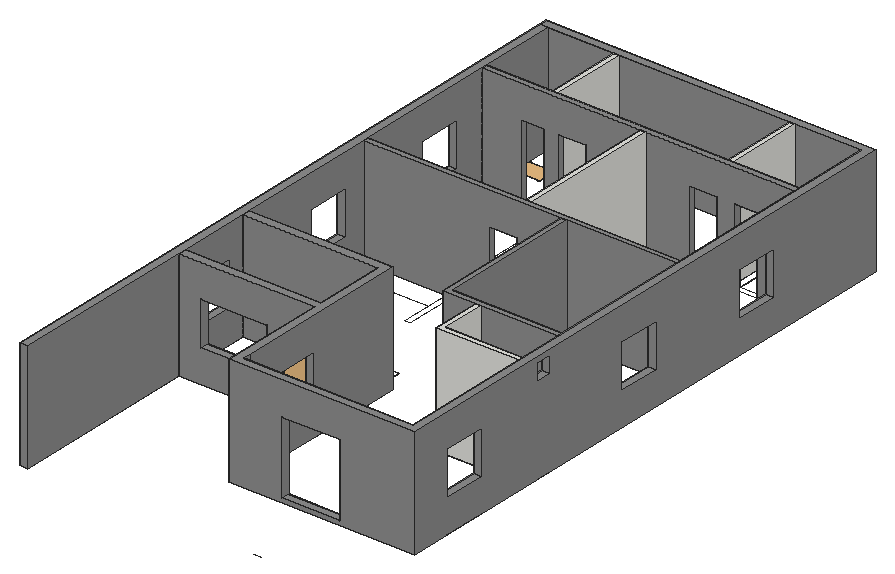
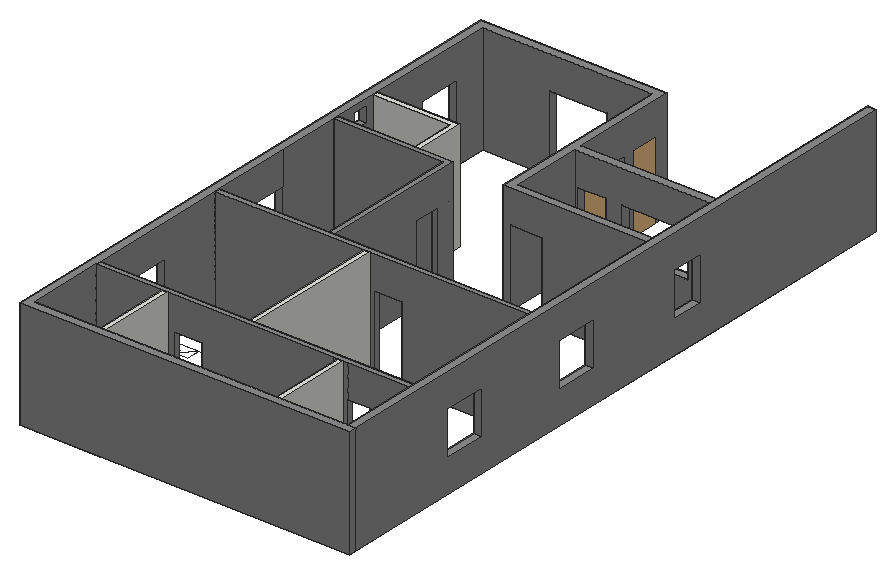
# SketchUp Ruby script. Lengths in inches.
U = 1.inch
M = Sketchup.active_model
def pt(a) = Geom::Point3d.new(a.map { |v| v * U })
def face(e, loops, mat)
  f = e.add_face(loops[0].map { |a| pt(a) })
  loops[1..].each { |l| e.add_face(l.map { |a| pt(a) }).erase! }
  f.material = f.back_material = mat if mat
  f
end
# faces: each face lists its corners as indices into pts; further lists are holes
def faces(e, pts, list, mat = nil) = list.each { |f| face(e, (f[0].is_a?(Array) ? f : [f]).map { |l| l.map { |i| pts[i] } }, mat) }
# xy, xz, yz: faces in a plane at the given z, y or x. An outline is a flat list of corners, or four numbers for a rectangle; further outlines are holes
def ring(l) = l.size == 4 ? [[l[0], l[1]], [l[2], l[1]], [l[2], l[3]], [l[0], l[3]]] : l.each_slice(2).to_a
def flat(e, list, mat, &to3) = list.each { |f| face(e, (f[0].is_a?(Array) ? f : [f]).map { |l| ring(l).map { |u, v| to3.(u, v) } }, mat) }
def xy(e, z, list, mat = nil) = flat(e, list, mat) { |x, y| [x, y, z] }
def xz(e, y, list, mat = nil) = flat(e, list, mat) { |x, z| [x, y, z] }
def yz(e, x, list, mat = nil) = flat(e, list, mat) { |y, z| [x, y, z] }
def lines(e, pts, list) = list.each { |a, b| e.add_line(pt(pts[a]), pt(pts[b])) }
# prism: a flat outline (further loops are holes) pulled along v
def prism(e, loops, v, mat = nil)
  f = face(e, loops, mat); d = Geom::Vector3d.new(v.map { |x| x * U })
  f.pushpull(f.normal.samedirection?(d) ? d.length : -d.length)
end
def box(e, o, s, mat = nil) = prism(e, [[o, [o[0] + s[0], o[1], o[2]], [o[0] + s[0], o[1] + s[1], o[2]], [o[0], o[1] + s[1], o[2]]]], [0, 0, s[2]], mat)
def at(x, y, z, deg = 0) = Geom::Transformation.translation(pt([x, y, z])) * Geom::Transformation.rotation(ORIGIN, Z_AXIS, deg.degrees)
def axes(o, x, y, z) = Geom::Transformation.new([*x, 0, *y, 0, *z, 0, *pt(o).to_a, 1])
def part(name) = M.definitions.add(name)
# library, detail: a bought-in or finely detailed component or shape, given as its bounding box
def library(name, o, s) = part(name).tap { |d| box(d.entities, o, s) }
def detail(e, o, s) = box(e.add_group.entities, o, s)
def put(e, d, t, mat = nil) = e.add_instance(d, t).tap { |i| i.material = mat if mat }
def group(e, t, mat = nil) = e.add_group.tap { |g| g.transformation = t; g.material = mat if mat }.entities
root = M.entities
M.materials.add("[Color M04]").color = [142, 142, 142]
c1 = library("PINTU 6 YA",[0,-0.6875,0],[35.83,8.07,80.71])
c2 = part("*U6")
p = [[-20,-17,0],[-20,23,0],[-18.25,23,0],[-18.25,-17,0],[20,-17,0],[19.92,-14.49,0],
  [19.68,-11.99,0],[19.29,-9.5,0],[18.74,-7.05,0],[18.04,-4.64,0],[17.19,-2.28,0],[16.19,0.03,0],
  [15.05,2.27,0],[13.77,4.43,0],[12.36,6.51,0],[10.82,8.5,0],[9.16,10.38,0],[7.38,12.16,0],
  [5.5,13.82,0],[3.51,15.36,0],[1.43,16.77,0],[-0.73,18.05,0],[-2.97,19.19,0],[-5.28,20.19,0],
  [-7.64,21.04,0],[-10.05,21.74,0],[-12.5,22.29,0],[-14.99,22.68,0],[-17.49,22.92,0],[-20,-23,0],
  [20,-23,0]]
lines(c2.entities,p,[[0,1],[1,2],[2,3],[3,0],[4,5],[5,6],[6,7],[7,8],[8,9],[9,10],[10,11],[11,12],
  [12,13],[13,14],[14,15],[15,16],[16,17],[17,18],[18,19],[19,20],[20,21],[21,22],[22,23],[23,24],
  [24,25],[25,26],[26,27],[27,28],[28,1],[0,29],[4,30]])
c3 = part("new block 03")
p = [[-4.5,18,0],[4.5,18,0],[4.5,-18,0],[-4.5,-18,0],[-1.33,-18,0],[-1.33,18,0],
  [1.57,18,0],[1.57,-18,0]]
lines(c3.entities,p,[[0,1],[1,2],[2,3],[3,0],[4,5],[5,6],[6,7]])
c4 = part("VENTILATOR")
p = [[-4.5,8.5,0],[4.5,8.5,0],[4.5,-8.5,0],[-4.5,-8.5,0],[0.58,8.5,0],[0.58,-8.5,0],
  [0,-8.5,0],[-1.15,-8.5,0],[-0.58,-8.5,0],[-0.58,8.5,0],[-1.15,8.5,0],[0,8.5,0]]
lines(c4.entities,p,[[0,1],[1,2],[2,3],[3,0],[4,5],[6,7],[8,9],[10,11]])
c5 = part("Bed - Queen")
p = [[22,23.6,0],[16.8,23.6,0],[22,38.8,0],[1.2,38.8,0],[1.2,25.6,0],[-1.2,38.8,0],
  [-1.2,25.6,0],[-22,38.8,0],[-22,25.6,0],[30,-40,0],[-30,-40,0],[-30,40,0],
  [14.8,23.2,0],[-30,23.2,0],[-30,25.6,0],[14.8,25.6,0],[30,40,0],[30,10.4,0],
  [14.8,10.4,0]]
lines(c5.entities,p,[[0,1],[2,0],[3,2],[4,3],[5,6],[7,5],[8,7],[9,10],[10,11],[12,13],[14,15],[11,16],
  [16,9],[17,15],[18,17],[15,18]])
c6 = library("*U4",[-21.75,-41.51,0],[21,28.01,0.01])
c7 = library("SINK",[-14.49,-22.42,0],[28.98,44.84,0.01])
c8 = part("new block 02")
p = [[-4.5,24,0],[4.5,24,0],[4.5,-24,0],[-4.5,-24,0],[-0.96,24,0],[-0.96,-24,0],
  [1.12,-24,0],[1.12,24,0]]
lines(c8.entities,p,[[0,1],[1,2],[2,3],[3,0],[4,5],[5,6],[6,7]])
c9 = part("Group14\#1")
box(c9.entities,[324.26,626,0],[6,84,120])
c10 = part("Group16\#1")
box(c10.entities,[132.26,626,0],[6,84,120])
c11 = part("Group20\#1")
box(c11.entities,[233.26,464,0],[6,156,120])
c12 = part("Group25\#1")
xy(c12.entities,0,[[312.3125,242,312.3125,265.39,318.3125,265.39,318.3125,248,402.3125,248,402.3125,242],[312.3125,289.39,318.3125,296]])
xy(c12.entities,84,[[312.3125,265.39,318.3125,289.39]])
xy(c12.entities,120,[[312.3125,242,402.3125,242,402.3125,248,318.3125,248,318.3125,296,312.3125,296]])
xz(c12.entities,242,[[312.3125,0,402.3125,120]])
xz(c12.entities,248,[[318.3125,0,402.3125,120]])
xz(c12.entities,265.39,[[312.3125,0,318.3125,84]])
xz(c12.entities,289.39,[[312.3125,0,318.3125,84]])
xz(c12.entities,296,[[312.3125,0,318.3125,120]])
yz(c12.entities,312.3125,[[242,0,242,120,296,120,296,0,289.39,0,289.39,84,265.39,84,265.39,0]])
yz(c12.entities,318.3125,[[248,0,265.39,0,265.39,84,289.39,84,289.39,0,296,0,296,120,248,120]])
yz(c12.entities,402.3125,[[242,0,248,120]])
p = [[11.9,753.72,126],[11.75,753.71,126],[14.46,751.33,126],[14.46,751.48,126],[14.44,751.64,126],[14.42,751.79,126],
  [14.38,751.95,126],[14.33,752.1,126],[14.28,752.25,126],[14.21,752.39,126],[14.14,752.53,126],[14.06,752.66,126],
  [13.97,752.79,126],[13.87,752.91,126],[13.76,753.02,126],[13.64,753.13,126],[13.52,753.23,126],[13.39,753.32,126],
  [13.26,753.41,126],[13.125,753.48,126],[12.98,753.54,126],[12.83,753.6,126],[12.68,753.65,126],[12.53,753.68,126],
  [12.375,753.71,126],[12.22,753.72,126],[12.0625,753.73,126],[11.59,753.68,126],[11.44,753.65,126],[11.29,753.6,126],
  [11.14,753.54,126],[11,753.48,126],[10.86,753.41,126],[10.73,753.32,126],[10.6,753.23,126],[10.48,753.13,126],
  [10.36,753.02,126],[10.26,752.91,126],[10.16,752.79,126],[10.07,752.66,126],[9.98,752.53,126],[9.91,752.39,126],
  [9.84,752.25,126],[9.79,752.1,126],[9.74,751.95,126],[9.71,751.79,126],[9.68,751.64,126],[9.67,751.48,126],
  [9.66,751.33,126],[9.67,751.17,126],[9.68,751.01,126],[9.71,750.86,126],[9.74,750.71,126],[9.79,750.55,126],
  [9.84,750.41,126],[9.91,750.26,126],[9.98,750.125,126],[10.07,749.99,126],[10.16,749.87,126],[10.26,749.74,126],
  [10.36,749.63,126],[10.48,749.52,126],[10.6,749.42,126],[10.73,749.33,126],[10.86,749.25,126],[11,749.17,126],
  [11.14,749.11,126],[11.29,749.05,126],[11.44,749.01,126],[11.59,748.97,126],[11.75,748.95,126],[11.9,748.93,126],
  [12.0625,748.93,126],[12.22,748.93,126],[12.375,748.95,126],[12.53,748.97,126],[12.68,749.01,126],[12.83,749.05,126],
  [12.98,749.11,126],[13.125,749.17,126],[13.26,749.25,126],[13.39,749.33,126],[13.52,749.42,126],[13.64,749.52,126],
  [13.76,749.63,126],[13.87,749.74,126],[13.97,749.87,126],[14.06,749.99,126],[14.14,750.125,126],[14.21,750.26,126],
  [14.28,750.41,126],[14.33,750.55,126],[14.38,750.71,126],[14.42,750.86,126],[14.44,751.01,126],[14.46,751.17,126],
  [166.65,162.5,126],[169.72,164.68,126],[166.65,167.26,126],[245.95,56.1875,120],[254.15,56.1875,120]]
lines(root,p,[[0,1],[2,3],[3,4],[4,5],[5,6],[6,7],[7,8],[8,9],[9,10],[10,11],[11,12],[12,13],
  [13,14],[14,15],[15,16],[16,17],[17,18],[18,19],[19,20],[20,21],[21,22],[22,23],[23,24],[24,25],
  [25,26],[26,0],[1,27],[27,28],[28,29],[29,30],[30,31],[31,32],[32,33],[33,34],[34,35],[35,36],
  [36,37],[37,38],[38,39],[39,40],[40,41],[41,42],[42,43],[43,44],[44,45],[45,46],[46,47],[47,48],
  [48,49],[49,50],[50,51],[51,52],[52,53],[53,54],[54,55],[55,56],[56,57],[57,58],[58,59],[59,60],
  [60,61],[61,62],[62,63],[63,64],[64,65],[65,66],[66,67],[67,68],[68,69],[69,70],[70,71],[71,72],
  [72,73],[73,74],[74,75],[75,76],[76,77],[77,78],[78,79],[79,80],[80,81],[81,82],[82,83],[83,84],
  [84,85],[85,86],[86,87],[87,88],[88,89],[89,90],[90,91],[91,92],[92,93],[93,94],[94,95],[95,2],
  [96,97],[98,96],[97,98],[99,100]])
put(root,c1,axes([157,179.85,126],[0,-0.82782,0],[1,0,0],[0,0,1.04078]))
put(root,c2,axes([64.02,677.99,126],[-0.6,0,0],[0,0.6,0],[0,0,0.6]))
put(root,c3,at(4.5,301.65,126))
put(root,c2,axes([297.72,677.99,126],[0.6,0,0],[0,0.6,0],[0,0,0.6]))
put(root,c4,at(355.55,308.92,126))
put(root,c5,axes([49,602.61,126],[0,-1,0],[-1,0,0],[0,0,1]))
put(root,c5,at(311.05,597.22,126,-90))
put(root,c2,axes([207.16,519.4375,126],[0.75,0,0],[0,0.75,0],[0,0,0.75]))
put(root,c6,at(326.59,767.6875,126))
put(root,c6,axes([332.8,278.6875,126],[1,0,0],[0,-1,0],[0,0,1]))
put(root,c4,at(334.46,758.6875,126,-90))
put(root,c2,axes([250.54,681.4375,126],[-0.75,0,0],[0,0.75,0],[0,0,0.75]))
put(root,c2,axes([107.56,681.4375,126],[0.75,0,0],[0,0.75,0],[0,0,0.75]))
put(root,c2,axes([161.57,519.4375,126],[-0.75,0,0],[0,0.75,0],[0,0,0.75]))
put(root,c6,at(-4.59,729.03,126,90.451))
put(root,c4,at(61.62,758.6875,126,-90))
put(root,c2,axes([174.25,165.1875,126],[0,0.75,0],[0.75,0,0],[0,0,0.75]))
put(root,c2,axes([242.3,376.49,126],[0,0.75,0],[0.75,0,0],[0,0,0.75]))
put(root,c7,axes([20.79,393.84,126],[0.70839,0,0],[0,0.70839,0],[0,0,0.70839]))
put(root,c2,axes([138.07,354.4375,126],[-0.75,0,0],[0,0.75,0],[0,0,0.75]))
put(root,c2,axes([138.49,267.4375,126],[-0.75,0,0],[0,0.75,0],[0,0,0.75]))
put(root,c8,at(355.55,201.2,126))
put(root,c5,at(311.05,430.19,126,-90))
put(root,c9,at(-51.26,44.1875,126))
put(root,c10,at(-51.26,44.1875,126))
put(root,c11,at(-51.26,44.1875,126))
put(root,c12,at(-51.26,44.1875,126))
g1 = group(root,at(0,44.1875,126),"[Color M04]")
xy(g1,0,[[0,0,9,239.47],[157,89,157,106,166,106,166,98,230.03,98,230.03,89],[230.03,89,278.03,92.38],[278.03,89,351.05,98],[351.05,89,360.05,371.28],
  [230.03,92.38,278.03,94.46],[230.03,94.46,278.03,98],[166,98,166.0625,106.25],[157,106,166,106.25],[157,135.66,157,136,166,135.66],
  [166,135.66,157,136,157,146.08,166,146.08],[157,146.08,160.54,146.14],[160.54,146.08,162.62,146.14],[162.62,146.08,166,146.14],[157,146.14,160.54,194.08],
  [160.54,146.14,162.62,194.08],[162.62,146.14,166,194.08],[157,194.08,166,206],[9,206,123.49,215],[153.49,206,157,215],
  [157,206,166,302],[0,239.47,9,385.56],[9,293,123.07,302],[225.05,296,351.05,302],[225.05,302,231.05,317.31],
  [225.05,347.31,231.05,458],[9,458,146.57,464],[176.57,458,192.16,464],[222.16,458,351.05,464],[351.05,532.1875,351.05,710,273,710,273,719,360.05,719,360.05,532.1875],
  [0,537.75,0,719,87,719,87,710,9,710,9,537.75],[9,620,52.02,626],[76.02,620,92.56,626],[122.56,620,235.54,626],[265.54,620,285.72,626],
  [309.72,620,351.05,626]])
xy(g1,4.3125,[[215.34,89,278.03,98]])
xy(g1,36,[[351.05,133.01,360.05,181.01],[157,146.14,166,194.25],[33,206,105,215],[0,239.47,9,275.35],[351.05,371.28,360.05,419.28],
  [0,385.56,9,433.56],[351.05,532.1875,360.05,580.1875],[0,537.75,9,585.75]])
xy(g1,84,[[215.34,89,278.03,98],[157,106.25,166,135.66],[351.05,133.01,360.05,181.01],[157,146.14,166,194.25],[33,206,105,215],
  [123.49,206,153.49,215],[0,239.47,9,275.35],[123.07,293,157,302],[225.05,317.31,231.05,347.31],[351.05,371.28,360.05,419.28],
  [0,385.56,9,433.56],[146.57,458,176.57,464],[192.16,458,222.16,464],[351.05,532.1875,360.05,580.1875],[0,537.75,9,585.75],
  [52.02,620,76.02,626],[92.56,620,122.56,626],[235.54,620,265.54,626],[285.72,620,309.72,626]])
xy(g1,96,[[351.05,256.23,360.05,274.23]])
xy(g1,114,[[351.05,256.23,360.05,274.23]])
xy(g1,120,[[0,0,9,710],[157,89,360.05,89,360.05,719,0,719,0,710,351.05,710,351.05,98,166.0625,98,166.0625,106.25,166,106.25,166,302,9,302,9,293,157,293,157,215,9,215,9,206,157,206],[225.05,296,351.05,296,351.05,302,231.05,302,231.05,458,225.05,458],[9,458,351.05,464],[9,620,351.05,626]])
xz(g1,0,[[0,0,9,120]])
xz(g1,89,[[[157,0,360.05,120],[215.34,4.3125,278.03,84]]])
xz(g1,98,[[[166.0625,0,351.05,120],[215.34,4.3125,278.03,84]]])
xz(g1,106.25,[[157,0,157,84,166,84,166,120,166.0625,120,166.0625,0]])
xz(g1,133.01,[[351.05,36,360.05,84]])
xz(g1,135.66,[[157,0,166,84]])
xz(g1,146.14,[[157,36,166,84]])
xz(g1,181.01,[[351.05,36,360.05,84]])
xz(g1,194.25,[[157,36,166,84]])
xz(g1,206,[[[9,0,123.49,0,123.49,84,153.49,84,153.49,0,157,0,157,120,9,120],[33,36,105,84]]])
xz(g1,215,[[[9,0,9,120,157,120,157,0,153.49,0,153.49,84,123.49,84,123.49,0],[33,36,105,84]]])
xz(g1,239.47,[[0,36,9,84]])
xz(g1,256.23,[[351.05,96,360.05,114]])
xz(g1,274.23,[[351.05,96,360.05,114]])
xz(g1,275.35,[[0,36,9,84]])
xz(g1,293,[[9,0,123.07,0,123.07,84,157,84,157,120,9,120]])
xz(g1,296,[[225.05,0,351.05,120]])
xz(g1,302,[[9,0,9,120,166,120,166,0,157,0,157,84,123.07,84,123.07,0],[231.05,0,351.05,120]])
xz(g1,317.31,[[225.05,0,231.05,84]])
xz(g1,347.31,[[225.05,0,231.05,84]])
xz(g1,371.28,[[351.05,36,360.05,84]])
xz(g1,385.56,[[0,36,9,84]])
xz(g1,419.28,[[351.05,36,360.05,84]])
xz(g1,433.56,[[0,36,9,84]])
xz(g1,458,[[9,0,146.57,0,146.57,84,176.57,84,176.57,0,192.16,0,192.16,84,222.16,84,222.16,0,225.05,0,225.05,120,9,120],[225.05,0,231.05,120],[231.05,0,351.05,120]])
xz(g1,464,[[9,0,9,120,351.05,120,351.05,0,222.16,0,222.16,84,192.16,84,192.16,0,176.57,0,176.57,84,146.57,84,146.57,0]])
xz(g1,532.1875,[[351.05,36,360.05,84]])
xz(g1,537.75,[[0,36,9,84]])
xz(g1,580.1875,[[351.05,36,360.05,84]])
xz(g1,585.75,[[0,36,9,84]])
xz(g1,620,[[9,0,52.02,0,52.02,84,76.02,84,76.02,0,92.56,0,92.56,84,122.56,84,122.56,0,235.54,0,235.54,84,265.54,84,265.54,0,285.72,0,285.72,84,309.72,84,309.72,0,351.05,0,351.05,120,9,120]])
xz(g1,626,[[9,0,9,120,76.02,120,76.02,84,52.02,84,52.02,0],[76.02,0,92.56,120],[122.56,0,122.56,84,92.56,84,92.56,120,351.05,120,351.05,0,309.72,0,309.72,84,285.72,84,285.72,0,265.54,0,265.54,84,235.54,84,235.54,0]])
xz(g1,710,[[9,0,351.05,120]])
xz(g1,719,[[0,0,360.05,120]])
yz(g1,0,[[[0,0,710,120],[537.75,36,585.75,84],[385.56,36,433.56,84],[239.47,36,275.35,84]],[710,0,719,120]])
yz(g1,9,[[0,0,206,120],[206,0,215,120],[[215,0,293,120],[239.47,36,275.35,84]],[293,0,302,120],[[302,0,458,120],[385.56,36,433.56,84]],
  [458,0,464,120],[[464,0,620,120],[537.75,36,585.75,84]],[620,0,626,120],[626,0,710,120]])
yz(g1,33,[[206,36,215,84]])
yz(g1,52.02,[[620,0,626,84]])
yz(g1,76.02,[[620,0,626,84]])
yz(g1,92.56,[[620,0,626,84]])
yz(g1,105,[[206,36,215,84]])
yz(g1,122.56,[[620,0,626,84]])
yz(g1,123.07,[[293,0,302,84]])
yz(g1,123.49,[[206,0,215,84]])
yz(g1,146.57,[[458,0,464,84]])
yz(g1,153.49,[[206,0,215,84]])
yz(g1,157,[[[89,0,89,120,206,120,206,0,135.66,0,135.66,84,106.25,84,106.25,0],[146.14,36,194.25,84]],[215,0,215,120,293,120,293,84,302,84,302,0]])
yz(g1,166,[[[135.66,0,302,0,302,120,106.25,120,106.25,84,135.66,84],[146.14,36,194.25,84]]])
yz(g1,166.0625,[[98,0,106.25,120]])
yz(g1,176.57,[[458,0,464,84]])
yz(g1,192.16,[[458,0,464,84]])
yz(g1,215.34,[[89,4.3125,98,84]])
yz(g1,222.16,[[458,0,464,84]])
yz(g1,225.05,[[296,0,296,120,458,120,458,0,347.31,0,347.31,84,317.31,84,317.31,0]])
yz(g1,231.05,[[302,0,317.31,0,317.31,84,347.31,84,347.31,0,458,0,458,120,302,120]])
yz(g1,235.54,[[620,0,626,84]])
yz(g1,265.54,[[620,0,626,84]])
yz(g1,278.03,[[89,4.3125,98,84]])
yz(g1,285.72,[[620,0,626,84]])
yz(g1,309.72,[[620,0,626,84]])
yz(g1,351.05,[[[98,0,296,120],[133.01,36,181.01,84],[256.23,96,274.23,114]],[296,0,302,120],[302,0,371.28,120],[371.28,0,371.28,36,419.28,36,419.28,84,371.28,84,371.28,120,458,120,458,0],[458,0,464,120],
  [[464,0,620,120],[532.1875,36,580.1875,84]],[620,0,626,120],[626,0,710,120]])
yz(g1,360.05,[[[89,0,719,120],[532.1875,36,580.1875,84],[133.01,36,181.01,84],[371.28,36,419.28,84],[256.23,96,274.23,114]]])
p = [[45,257,0],[45,293,0],[222.13,464,0],[222.16,464,0],[261.05,296,0],[261.05,242,0],
  [267.05,248,0],[351.05,248,0],[153.07,302,0],[157,302,0],[182,620,0],[182,464,0],
  [105.05,353.74,0],[105.05,302,0],[351.05,242,0],[188,620,0],[188,464,0],[81,710,0],
  [81,626,0],[273,710,0],[273,626,0],[9,257,0],[9,251,0],[45,251,0],
  [87,710,0],[87,626,0],[267.05,296,0],[166,107.3125,0],[166,106.25,0],[279,710,0],
  [279,626,0],[75,257,0],[75,293,0],[99,458,0],[99,434,0],[99,353.74,0],
  [99,302,0],[105.05,458,0],[105.05,401.74,0],[122.52,626,0],[122.56,626,0],[105,251,0],
  [105,232.1875,0],[65,257,0],[65,293,0],[85,257,0],[85,293,0],[65,251,0],
  [65,232.1875,0],[37.2,234.69,0],[37.2,232.1875,0],[37.2,229.73,0],[33.94,232.1875,0],[55,257,0],
  [55,293,0],[85,251,0],[85,232.1875,0],[71.09,229.73,0],[67.84,232.1875,0],[95,257,0],
  [95,293,0],[71.09,234.69,0],[71.09,232.1875,0],[95,251,0],[95,232.1875,0],[115,251,0],
  [115,257,0],[75,251,0],[75,232.1875,0],[117.74,232.1875,0],[55,251,0],[55,232.1875,0],
  [231.05,302,84],[225.05,302,84],[153.07,293,0],[157,293,0],[222.16,458,0],[105,257,0],
  [105,293,0],[45,232.1875,0],[44.11,434,0],[44.11,302,0],[99,401.74,0],[75,215,0],
  [122.52,620,0],[123.49,215,0],[123.83,215,0],[65,215,0],[95,215,0],[231.05,347.31,0],
  [231.05,347.27,0],[105,215,0],[146.57,464,0],[146.61,464,0],[52.02,620,0],[76.02,620,0],
  [123.49,206,0],[153.49,206,0],[45,215,0],[122.56,620,0],[34.15,232.1875,0],[235.54,626,0],
  [235.58,626,0],[115,293,0],[225.05,347.31,0],[225.05,317.31,0],[123.07,302,0],[123.41,302,0],
  [85,215,0],[55,215,0],[192.16,458,0],[123.07,293,0],[146.57,458,0],[176.57,458,0],
  [235.54,620,0],[265.54,620,0],[157,135.66,0],[157,106.25,0],[285.72,626,0],[309.72,626,0],
  [92.56,620,0],[285.72,620,0],[309.72,620,0]]
lines(g1,p,[[0,1],[2,3],[4,5],[6,7],[8,9],[10,11],[12,13],[5,14],[15,16],[17,18],[19,20],[21,0],
  [22,23],[24,25],[26,6],[27,28],[29,30],[31,32],[33,34],[35,36],[37,38],[39,40],[41,42],[43,44],
  [45,46],[47,48],[49,50],[51,52],[53,54],[55,56],[57,58],[59,60],[52,49],[61,62],[63,64],[65,66],
  [67,68],[69,42],[70,71],[72,73],[12,35],[74,75],[76,2],[77,78],[23,79],[58,61],[80,81],[82,38],
  [34,80],[31,45],[63,41],[0,53],[56,68],[42,64],[68,83],[39,84],[85,86],[48,87],[64,88],[62,58],
  [74,8],[89,90],[42,91],[23,70],[92,93],[62,57],[50,51],[94,95],[96,97],[79,98],[84,99],[67,55],
  [58,48],[50,100],[101,102],[66,103],[48,71],[79,50],[71,79],[64,56],[104,105],[45,59],[43,31],[106,107],
  [56,108],[71,109],[34,82],[68,62],[110,76],[53,43],[47,67],[111,74],[41,65],[112,113],[114,115],[59,77],
  [55,63],[77,66],[116,117],[70,47],[118,119],[120,84],[121,122]])
put(root,c1,axes([123.49,250.25,126],[0.83729,0,0],[0,0.08537,0],[0,0,1.04078]))
